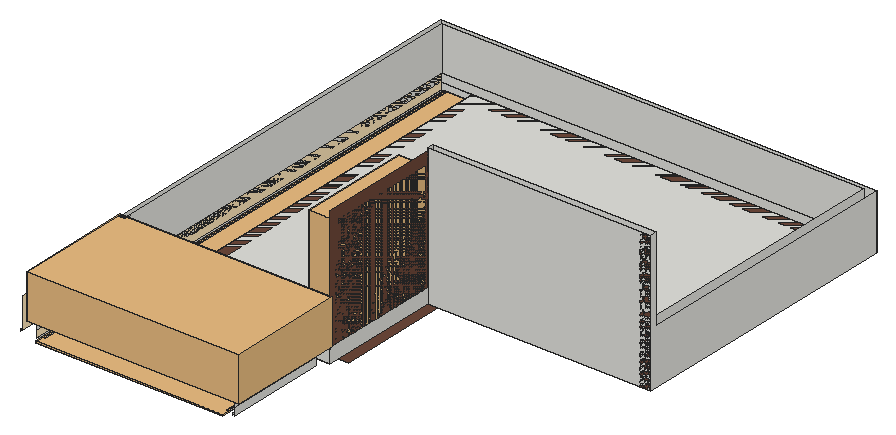
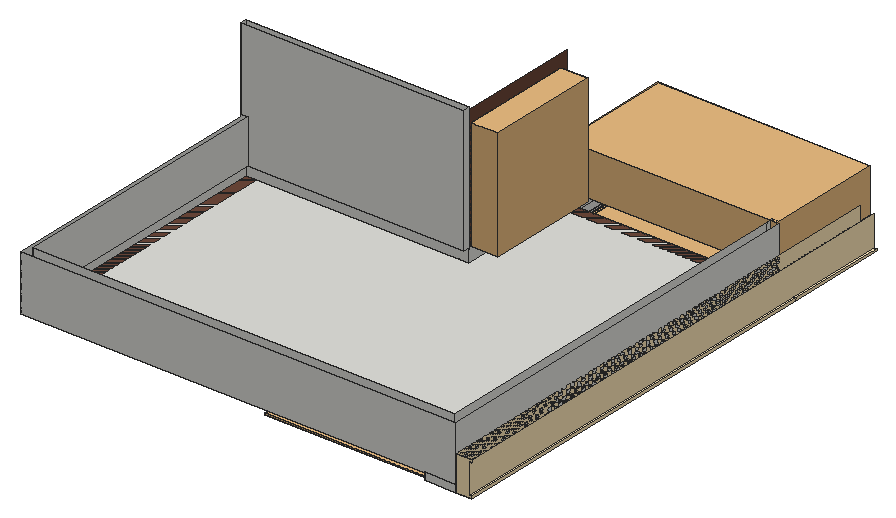
# SketchUp Ruby script. Lengths in inches.
U = 1.inch
M = Sketchup.active_model
def pt(a) = Geom::Point3d.new(a.map { |v| v * U })
def face(e, loops, mat)
  f = e.add_face(loops[0].map { |a| pt(a) })
  loops[1..].each { |l| e.add_face(l.map { |a| pt(a) }).erase! }
  f.material = f.back_material = mat if mat
  f
end
# faces: each face lists its corners as indices into pts; further lists are holes
def faces(e, pts, list, mat = nil) = list.each { |f| face(e, (f[0].is_a?(Array) ? f : [f]).map { |l| l.map { |i| pts[i] } }, mat) }
# xy, xz, yz: faces in a plane at the given z, y or x. An outline is a flat list of corners, or four numbers for a rectangle; further outlines are holes
def ring(l) = l.size == 4 ? [[l[0], l[1]], [l[2], l[1]], [l[2], l[3]], [l[0], l[3]]] : l.each_slice(2).to_a
def flat(e, list, mat, &to3) = list.each { |f| face(e, (f[0].is_a?(Array) ? f : [f]).map { |l| ring(l).map { |u, v| to3.(u, v) } }, mat) }
def xy(e, z, list, mat = nil) = flat(e, list, mat) { |x, y| [x, y, z] }
def xz(e, y, list, mat = nil) = flat(e, list, mat) { |x, z| [x, y, z] }
def yz(e, x, list, mat = nil) = flat(e, list, mat) { |y, z| [x, y, z] }
def lines(e, pts, list) = list.each { |a, b| e.add_line(pt(pts[a]), pt(pts[b])) }
# prism: a flat outline (further loops are holes) pulled along v
def prism(e, loops, v, mat = nil)
  f = face(e, loops, mat); d = Geom::Vector3d.new(v.map { |x| x * U })
  f.pushpull(f.normal.samedirection?(d) ? d.length : -d.length)
end
def box(e, o, s, mat = nil) = prism(e, [[o, [o[0] + s[0], o[1], o[2]], [o[0] + s[0], o[1] + s[1], o[2]], [o[0], o[1] + s[1], o[2]]]], [0, 0, s[2]], mat)
def at(x, y, z, deg = 0) = Geom::Transformation.translation(pt([x, y, z])) * Geom::Transformation.rotation(ORIGIN, Z_AXIS, deg.degrees)
def axes(o, x, y, z) = Geom::Transformation.new([*x, 0, *y, 0, *z, 0, *pt(o).to_a, 1])
def part(name) = M.definitions.add(name)
# library, detail: a bought-in or finely detailed component or shape, given as its bounding box
def library(name, o, s) = part(name).tap { |d| box(d.entities, o, s) }
def detail(e, o, s) = box(e.add_group.entities, o, s)
def put(e, d, t, mat = nil) = e.add_instance(d, t).tap { |i| i.material = mat if mat }
def group(e, t, mat = nil) = e.add_group.tap { |g| g.transformation = t; g.material = mat if mat }.entities
root = M.entities
M.materials.add("1026 AP 7946 SUNNY SIDE UP").color = [254, 231, 186]
M.materials.add("1916 AP K226 Macadamia Cream-N").color = [109, 72, 58]
M.materials.add("False Ceiling Light").color = [254, 233, 206]
M.materials.add("[Steel Brushed Stainless]").color = [48, 48, 48]
c1 = library("Group\#24",[0,0,0],[182.5,101,38])
c2 = library("Vertical garden rack",[-1.0625,86.33,0],[73.76,23.18,83.06])
c3 = library("Group\#55",[0,0,0],[161,440,1])
xy(root,246,[[4,325.996,6,326,18,326],[4,326,18,674]],"1026 AP 7946 SUNNY SIDE UP")
xy(root,248,[[6.162,238.937,6,326,5.775,326,4.742,325.998,4.162,325.996,4,325.996,4.162,238.948],[4.162,325.996,4.742,325.998,5.775,326,4.162,326],[4,326,6,674]],"1026 AP 7946 SUNNY SIDE UP")
xy(root,252,[[45,325.75,45,674,393,674,393,431,201,431,201,326,189,326,189,325.75]])
xy(root,252,[[45,326,201,326,201,335,54,335,54,665,384,665,384,431,393,431,393,674,45,674],[201,335,210,431]],"1916 AP K226 Macadamia Cream-N")
xz(root,323.75,[[43,246,182,247],[182,246,184,248],[184,246,186.945,247],[186.945,246,187,247]])
xz(root,325.75,[[45,246,189,252]])
xz(root,326,[[189,252,201,264]])
xz(root,326,[[4,246,6,248]],"1026 AP 7946 SUNNY SIDE UP")
xz(root,326.094,[[18,264,24,302]])
xz(root,431,[[201,252,393,372]])
xz(root,431,[[201,252,210,372],[384,252,393,372]],"1916 AP K226 Macadamia Cream-N")
xz(root,437,[[201,264,201,372,393,372,393,302,387,302,387,264]])
xz(root,668,[[24,264,387,302]])
xz(root,672,[[20,246,23,247],[23,246,25,248],[25,246,43,247]])
xz(root,674,[[18,246,45,252],[18,252,393,300]])
xz(root,674,[[4,246,4,248,6,248,6,274,4,274,4,276,18,276,18,246]],"1026 AP 7946 SUNNY SIDE UP")
yz(root,4,[[326,246,674,248]],"1026 AP 7946 SUNNY SIDE UP")
yz(root,6,[[239,248,674,274]],"1026 AP 7946 SUNNY SIDE UP")
yz(root,18,[[239,246,674,252],[239,252,239,264,326.094,264,326.094,300,674,300,674,252]])
yz(root,18,[[239,246,674,276]],"1026 AP 7946 SUNNY SIDE UP")
yz(root,20,[[239,246,672,247]])
yz(root,23,[[239,247,672,248]])
yz(root,24,[[326.094,264,332.094,302],[332.094,264,668,302]])
yz(root,25,[[239,247,672,248]])
yz(root,43,[[323.75,246,672,247]])
yz(root,45,[[325.75,246,674,252]])
yz(root,182,[[239,247,323.75,248]])
yz(root,184,[[239,247,323.75,248]])
yz(root,187,[[239,246,323.75,247]])
yz(root,189,[[239,246,325.75,252],[239,252,326,264]])
yz(root,201,[[326,252,431,264],[431,264,437,372]])
yz(root,201,[[326,252,431,370]],"1916 AP K226 Macadamia Cream-N")
yz(root,387,[[437,264,668,302]])
yz(root,393,[[431,252,674,252,674,300,437,300,437,372,431,372]])
p = [[4,325.996,246],[4.162,238.948,246],[4.162,238.948,248],[4,325.996,248],[4.162,325.996,248],[4.742,325.998,248],
  [5.775,326,248],[5.838,326,248],[6,326,248],[6,326,246],[53.497,277.317,250],[53.497,277.317,247],
  [53.539,277.384,247],[53.539,277.384,250],[58.613,277.317,250],[58.613,277.317,247],[58.653,277.25,247],[58.653,277.25,250],
  [58.571,277.384,250],[58.571,277.384,247],[100.942,277.317,250],[100.942,277.317,247],[100.984,277.384,247],[100.984,277.384,250],
  [106.016,277.384,250],[106.016,277.384,247],[106.058,277.317,247],[106.058,277.317,250],[148.387,277.317,250],[148.387,277.317,247],
  [148.429,277.384,247],[148.429,277.384,250],[153.461,277.384,250],[153.461,277.384,247],[153.503,277.317,247],[153.503,277.317,250],
  [53.582,277.449,247],[53.582,277.449,250],[53.628,277.513,247],[53.628,277.513,250],[58.527,277.449,250],[58.527,277.449,247],
  [58.482,277.513,250],[58.482,277.513,247],[101.028,277.449,247],[101.028,277.449,250],[101.073,277.513,247],[101.073,277.513,250],
  [105.927,277.513,250],[105.927,277.513,247],[105.972,277.449,247],[105.972,277.449,250],[148.473,277.449,247],[148.473,277.449,250],
  [148.518,277.513,247],[148.518,277.513,250],[153.418,277.449,250],[153.418,277.449,247],[153.372,277.513,250],[153.372,277.513,247],
  [53.675,277.576,247],[53.675,277.576,250],[58.435,277.576,250],[58.435,277.576,247],[101.12,277.576,247],[101.12,277.576,250],
  [105.88,277.576,250],[105.88,277.576,247],[148.565,277.576,247],[148.565,277.576,250],[153.325,277.576,250],[153.325,277.576,247],
  [53.723,277.638,247],[53.723,277.638,250],[53.774,277.698,247],[53.774,277.698,250],[58.336,277.698,250],[58.336,277.698,247],
  [58.386,277.638,247],[58.386,277.638,250],[101.169,277.638,247],[101.169,277.638,250],[101.219,277.698,247],[101.219,277.698,250],
  [105.831,277.638,250],[105.831,277.638,247],[105.781,277.698,250],[105.781,277.698,247],[148.614,277.638,247],[148.614,277.638,250],
  [148.664,277.698,247],[148.664,277.698,250],[153.226,277.698,250],[153.226,277.698,247],[153.277,277.638,247],[153.277,277.638,250],
  [53.825,277.757,247],[53.825,277.757,250],[58.284,277.757,250],[58.284,277.757,247],[101.271,277.757,247],[101.271,277.757,250],
  [105.729,277.757,250],[105.729,277.757,247],[148.716,277.757,247],[148.716,277.757,250],[153.175,277.757,250],[153.175,277.757,247],
  [53.879,277.815,247],[53.879,277.815,250],[53.933,277.871,247],[53.933,277.871,250],[58.231,277.815,250],[58.231,277.815,247],
  [58.176,277.871,250],[58.176,277.871,247],[101.324,277.815,247],[101.324,277.815,250],[101.379,277.871,247],[101.379,277.871,250],
  [105.621,277.871,250],[105.621,277.871,247],[105.676,277.815,247],[105.676,277.815,250],[148.769,277.815,247],[148.769,277.815,250],
  [148.824,277.871,247],[148.824,277.871,250],[153.121,277.815,250],[153.121,277.815,247],[153.067,277.871,250],[153.067,277.871,247],
  [53.99,277.926,247],[53.99,277.926,250],[54.047,277.979,247],[54.047,277.979,250],[58.12,277.926,250],[58.12,277.926,247],
  [58.062,277.979,250],[58.062,277.979,247],[101.435,277.926,247],[101.435,277.926,250],[101.493,277.979,247],[101.493,277.979,250],
  [105.507,277.979,250],[105.507,277.979,247],[105.565,277.926,247],[105.565,277.926,250],[148.88,277.926,247],[148.88,277.926,250],
  [148.938,277.979,247],[148.938,277.979,250],[153.01,277.926,250],[153.01,277.926,247],[152.953,277.979,250],[152.953,277.979,247],
  [54.106,278.031,247],[54.106,278.031,250],[54.167,278.081,247],[54.167,278.081,250],[57.943,278.081,250],[57.943,278.081,247],
  [58.003,278.031,247],[58.003,278.031,250],[101.552,278.031,247],[101.552,278.031,250],[101.612,278.081,247],[101.612,278.081,250],
  [105.448,278.031,250],[105.448,278.031,247],[105.388,278.081,250],[105.388,278.081,247],[148.997,278.031,247],[148.997,278.031,250],
  [149.057,278.081,247],[149.057,278.081,250],[152.833,278.081,250],[152.833,278.081,247],[152.894,278.031,247],[152.894,278.031,250],
  [54.228,278.13,247],[54.228,278.13,250],[54.291,278.177,247],[54.291,278.177,250],[57.818,278.177,250],[57.818,278.177,247],
  [57.881,278.13,247],[57.881,278.13,250],[101.674,278.13,247],[101.674,278.13,250],[101.737,278.177,247],[101.737,278.177,250],
  [105.326,278.13,250],[105.326,278.13,247],[105.263,278.177,250],[105.263,278.177,247],[149.119,278.13,247],[149.119,278.13,250],
  [149.182,278.177,247],[149.182,278.177,250],[152.709,278.177,250],[152.709,278.177,247],[152.772,278.13,247],[152.772,278.13,250],
  [54.356,278.222,247],[54.356,278.222,250],[54.421,278.266,247],[54.421,278.266,250],[57.689,278.266,250],[57.689,278.266,247],
  [57.754,278.222,247],[57.754,278.222,250],[101.801,278.222,247],[101.801,278.222,250],[101.866,278.266,247],[101.866,278.266,250],
  [105.134,278.266,250],[105.134,278.266,247],[105.199,278.222,247],[105.199,278.222,250],[149.246,278.222,247],[149.246,278.222,250],
  [149.311,278.266,247],[149.311,278.266,250],[152.644,278.222,250],[152.644,278.222,247],[152.579,278.266,250],[152.579,278.266,247],
  [54.487,278.308,247],[54.487,278.308,250],[54.555,278.348,247],[54.555,278.348,250],[54.623,278.386,247],[54.623,278.386,250],
  [57.486,278.386,250],[57.486,278.386,247],[57.555,278.348,247],[57.555,278.348,250],[57.622,278.308,250],[57.622,278.308,247],
  [101.933,278.308,247],[101.933,278.308,250],[102,278.348,247],[102,278.348,250],[102.069,278.386,247],[102.069,278.386,250],
  [104.931,278.386,250],[104.931,278.386,247],[105,278.348,247],[105,278.348,250],[105.067,278.308,247],[105.067,278.308,250],
  [149.378,278.308,247],[149.378,278.308,250],[149.445,278.348,247],[149.445,278.348,250],[149.514,278.386,247],[149.514,278.386,250],
  [152.445,278.348,250],[152.445,278.348,247],[152.513,278.308,247],[152.513,278.308,250],[152.377,278.386,250],[152.377,278.386,247],
  [54.693,278.423,247],[54.693,278.423,250],[54.763,278.458,247],[54.763,278.458,250],[57.346,278.458,250],[57.346,278.458,247],
  [57.417,278.423,247],[57.417,278.423,250],[102.138,278.423,247],[102.138,278.423,250],[102.208,278.458,247],[102.208,278.458,250],
  [104.792,278.458,250],[104.792,278.458,247],[104.862,278.423,247],[104.862,278.423,250],[149.583,278.423,247],[149.583,278.423,250],
  [149.654,278.458,247],[149.654,278.458,250],[152.237,278.458,250],[152.237,278.458,247],[152.307,278.423,247],[152.307,278.423,250],
  [54.835,278.491,247],[54.835,278.491,250],[54.907,278.522,247],[54.907,278.522,250],[54.98,278.551,247],[54.98,278.551,250],
  [57.13,278.551,250],[57.13,278.551,247],[57.203,278.522,247],[57.203,278.522,250],[57.275,278.491,247],[57.275,278.491,250],
  [102.28,278.491,247],[102.28,278.491,250],[102.352,278.522,247],[102.352,278.522,250],[102.425,278.551,247],[102.425,278.551,250],
  [104.648,278.522,250],[104.648,278.522,247],[104.72,278.491,247],[104.72,278.491,250],[104.575,278.551,250],[104.575,278.551,247],
  [149.725,278.491,247],[149.725,278.491,250],[149.797,278.522,247],[149.797,278.522,250],[149.87,278.551,247],[149.87,278.551,250],
  [152.02,278.551,250],[152.02,278.551,247],[152.093,278.522,247],[152.093,278.522,250],[152.165,278.491,247],[152.165,278.491,250],
  [55.053,278.578,247],[55.053,278.578,250],[55.128,278.603,247],[55.128,278.603,250],[55.203,278.626,247],[55.203,278.626,250],
  [55.278,278.648,247],[55.278,278.648,250],[55.354,278.667,247],[55.354,278.667,250],[56.831,278.648,250],[56.831,278.648,247],
  [56.907,278.626,247],[56.907,278.626,250],[56.755,278.667,250],[56.755,278.667,247],[56.982,278.603,247],[56.982,278.603,250],
  [57.056,278.578,247],[57.056,278.578,250],[102.499,278.578,247],[102.499,278.578,250],[102.573,278.603,247],[102.573,278.603,250],
  [102.648,278.626,247],[102.648,278.626,250],[102.724,278.648,247],[102.724,278.648,250],[102.8,278.667,247],[102.8,278.667,250],
  [104.2,278.667,250],[104.2,278.667,247],[104.276,278.648,247],[104.276,278.648,250],[104.352,278.626,247],[104.352,278.626,250],
  [104.427,278.603,250],[104.427,278.603,247],[104.501,278.578,247],[104.501,278.578,250],[149.944,278.578,247],[149.944,278.578,250],
  [150.018,278.603,247],[150.018,278.603,250],[150.093,278.626,247],[150.093,278.626,250],[150.169,278.648,247],[150.169,278.648,250],
  [150.245,278.667,247],[150.245,278.667,250],[151.646,278.667,250],[151.646,278.667,247],[151.722,278.648,247],[151.722,278.648,250],
  [151.797,278.626,247],[151.797,278.626,250],[151.872,278.603,247],[151.872,278.603,250],[151.947,278.578,250],[151.947,278.578,247],
  [55.431,278.684,247],[55.431,278.684,250],[55.508,278.7,247],[55.508,278.7,250],[55.585,278.713,247],[55.585,278.713,250],
  [55.663,278.724,247],[55.663,278.724,250],[55.741,278.734,247],[55.741,278.734,250],[55.819,278.741,247],[55.819,278.741,250],
  [55.898,278.746,247],[55.898,278.746,250],[55.976,278.749,247],[55.976,278.749,250],[56.055,278.75,247],[56.055,278.75,250],
  [56.133,278.749,250],[56.133,278.749,247],[56.212,278.746,247],[56.212,278.746,250],[56.29,278.741,247],[56.29,278.741,250],
  [56.368,278.734,247],[56.368,278.734,250],[56.446,278.724,250],[56.446,278.724,247],[56.524,278.713,247],[56.524,278.713,250],
  [56.601,278.7,247],[56.601,278.7,250],[56.679,278.684,247],[56.679,278.684,250],[102.876,278.684,247],[102.876,278.684,250],
  [102.953,278.7,247],[102.953,278.7,250],[103.031,278.713,247],[103.031,278.713,250],[103.108,278.724,247],[103.108,278.724,250],
  [103.186,278.734,247],[103.186,278.734,250],[103.265,278.741,247],[103.265,278.741,250],[103.343,278.746,247],[103.343,278.746,250],
  [103.421,278.749,247],[103.421,278.749,250],[103.5,278.75,247],[103.5,278.75,250],[103.579,278.749,247],[103.579,278.749,250],
  [103.657,278.746,247],[103.657,278.746,250],[103.735,278.741,250],[103.735,278.741,247],[103.814,278.734,247],[103.814,278.734,250],
  [103.892,278.724,247],[103.892,278.724,250],[103.969,278.713,247],[103.969,278.713,250],[104.047,278.7,250],[104.047,278.7,247],
  [104.124,278.684,247],[104.124,278.684,250],[150.321,278.684,247],[150.321,278.684,250],[150.399,278.7,247],[150.399,278.7,250],
  [150.476,278.713,247],[150.476,278.713,250],[150.554,278.724,247],[150.554,278.724,250],[150.632,278.734,247],[150.632,278.734,250],
  [150.71,278.741,247],[150.71,278.741,250],[150.788,278.746,247],[150.788,278.746,250],[150.867,278.749,247],[150.867,278.749,250],
  [150.945,278.75,247],[150.945,278.75,250],[151.024,278.749,247],[151.024,278.749,250],[151.102,278.746,247],[151.102,278.746,250],
  [151.181,278.741,247],[151.181,278.741,250],[151.259,278.734,247],[151.259,278.734,250],[151.337,278.724,250],[151.337,278.724,247],
  [151.415,278.713,247],[151.415,278.713,250],[151.492,278.7,247],[151.492,278.7,250],[151.569,278.684,247],[151.569,278.684,250],
  [186.945,323.75,246],[186.945,239,246]]
faces(root,p,[[0,1,2,3],[3,4,5,6,7,8,9,0]],"1026 AP 7946 SUNNY SIDE UP")
faces(root,p,[[10,11,12,13],[14,15,16,17],[18,19,15,14],[20,21,22,23],[24,25,26,27],[28,29,30,31],[32,33,34,35],[13,12,36,37],
  [37,36,38,39],[40,41,19,18],[42,43,41,40],[23,22,44,45],[45,44,46,47],[48,49,50,51],[51,50,25,24],[31,30,52,53],
  [53,52,54,55],[56,57,33,32],[58,59,57,56],[39,38,60,61],[62,63,43,42],[47,46,64,65],[66,67,49,48],[55,54,68,69],
  [70,71,59,58],[61,60,72,73],[73,72,74,75],[76,77,78,79],[79,78,63,62],[65,64,80,81],[81,80,82,83],[84,85,67,66],
  [86,87,85,84],[69,68,88,89],[89,88,90,91],[92,93,94,95],[95,94,71,70],[75,74,96,97],[98,99,77,76],[83,82,100,101],
  [102,103,87,86],[91,90,104,105],[106,107,93,92],[97,96,108,109],[109,108,110,111],[112,113,99,98],[114,115,113,112],[101,100,116,117],
  [117,116,118,119],[120,121,122,123],[123,122,103,102],[105,104,124,125],[125,124,126,127],[128,129,107,106],[130,131,129,128],[111,110,132,133],
  [133,132,134,135],[136,137,115,114],[138,139,137,136],[119,118,140,141],[141,140,142,143],[144,145,146,147],[147,146,121,120],[127,126,148,149],
  [149,148,150,151],[152,153,131,130],[154,155,153,152],[135,134,156,157],[157,156,158,159],[160,161,162,163],[163,162,139,138],[143,142,164,165],
  [165,164,166,167],[168,169,145,144],[170,171,169,168],[151,150,172,173],[173,172,174,175],[176,177,178,179],[179,178,155,154],[159,158,180,181],
  [181,180,182,183],[184,185,186,187],[187,186,161,160],[167,166,188,189],[189,188,190,191],[192,193,171,170],[194,195,193,192],[175,174,196,197],
  [197,196,198,199],[200,201,202,203],[203,202,177,176],[183,182,204,205],[205,204,206,207],[208,209,210,211],[211,210,185,184],[191,190,212,213],
  [213,212,214,215],[216,217,218,219],[219,218,195,194],[199,198,220,221],[221,220,222,223],[224,225,201,200],[226,227,225,224],[207,206,228,229],
  [229,228,230,231],[231,230,232,233],[234,235,236,237],[238,239,209,208],[237,236,239,238],[215,214,240,241],[241,240,242,243],[243,242,244,245],
  [246,247,248,249],[249,248,250,251],[251,250,217,216],[223,222,252,253],[253,252,254,255],[255,254,256,257],[258,259,260,261],[262,263,259,258],
  [261,260,227,226],[233,232,264,265],[265,264,266,267],[268,269,270,271],[271,270,235,234],[245,244,272,273],[273,272,274,275],[276,277,278,279],
  [279,278,247,246],[257,256,280,281],[281,280,282,283],[284,285,286,287],[287,286,263,262],[267,266,288,289],[289,288,290,291],[291,290,292,293],
  [294,295,296,297],[297,296,298,299],[299,298,269,268],[275,274,300,301],[301,300,302,303],[303,302,304,305],[306,307,308,309],[310,311,307,306],
  [309,308,277,276],[283,282,312,313],[313,312,314,315],[315,314,316,317],[318,319,320,321],[321,320,322,323],[323,322,285,284],[293,292,324,325],
  [325,324,326,327],[327,326,328,329],[329,328,330,331],[331,330,332,333],[334,335,336,337],[338,339,335,334],[337,336,340,341],[341,340,342,343],
  [343,342,295,294],[305,304,344,345],[345,344,346,347],[347,346,348,349],[349,348,350,351],[351,350,352,353],[354,355,356,357],[357,356,358,359],
  [360,361,362,363],[359,358,361,360],[363,362,311,310],[317,316,364,365],[365,364,366,367],[367,366,368,369],[369,368,370,371],[371,370,372,373],
  [374,375,376,377],[377,376,378,379],[379,378,380,381],[382,383,319,318],[381,380,383,382],[333,332,384,385],[385,384,386,387],[387,386,388,389],
  [389,388,390,391],[391,390,392,393],[393,392,394,395],[395,394,396,397],[397,396,398,399],[399,398,400,401],[402,403,404,405],[401,400,403,402],
  [405,404,406,407],[407,406,408,409],[410,411,412,413],[409,408,411,410],[413,412,414,415],[415,414,416,417],[417,416,339,338],[353,352,418,419],
  [419,418,420,421],[421,420,422,423],[423,422,424,425],[425,424,426,427],[427,426,428,429],[429,428,430,431],[431,430,432,433],[433,432,434,435],
  [435,434,436,437],[437,436,438,439],[440,441,442,443],[439,438,441,440],[443,442,444,445],[445,444,446,447],[448,449,450,451],[447,446,449,448],
  [451,450,355,354],[373,372,452,453],[453,452,454,455],[455,454,456,457],[457,456,458,459],[459,458,460,461],[461,460,462,463],[463,462,464,465],
  [465,464,466,467],[467,466,468,469],[469,468,470,471],[471,470,472,473],[473,472,474,475],[475,474,476,477],[478,479,480,481],[477,476,479,478],
  [481,480,482,483],[483,482,484,485],[485,484,375,374]])
lines(root,p,[[486,487]])
put(root,c1,at(18.5,227.5,264),"[Steel Brushed Stainless]")
put(root,c2,axes([91.49,427.7,264],[0,-1.31,0],[1,0,0],[0,0,1.15]),"1026 AP 7946 SUNNY SIDE UP")
put(root,c3,at(23,232,247),"False Ceiling Light")
